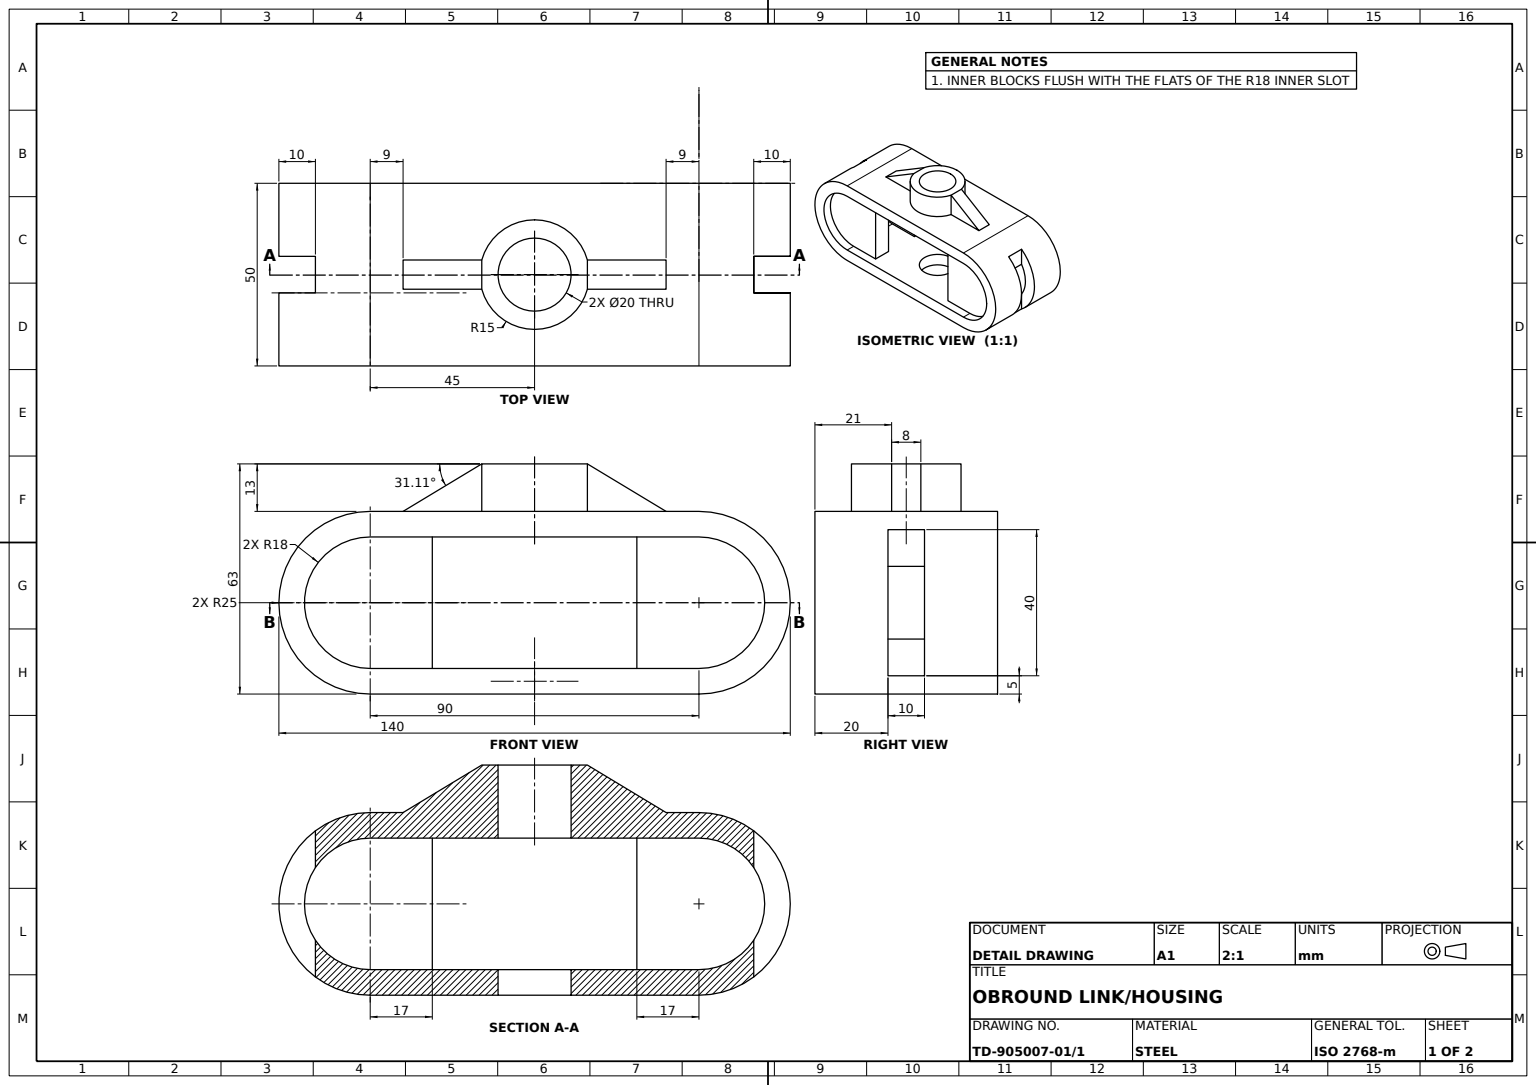
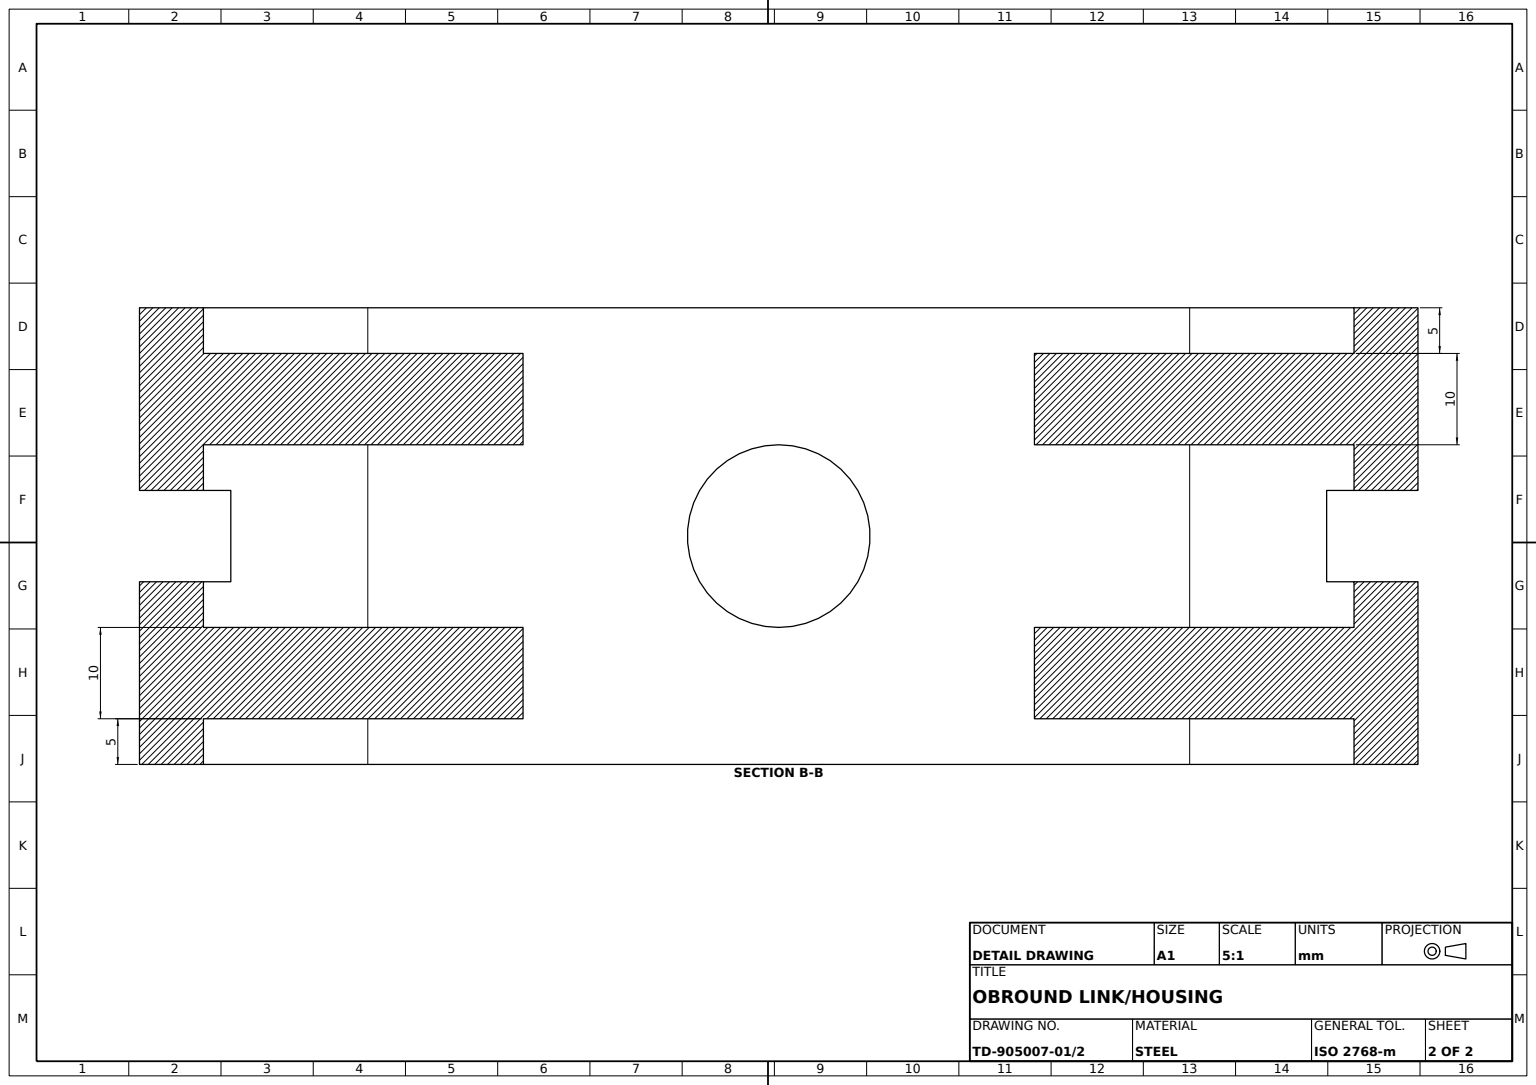
ISO-10303-21;
HEADER;
FILE_DESCRIPTION((''),'2;1');
FILE_NAME('','',(''),(''),'','','');
FILE_SCHEMA(('AUTOMOTIVE_DESIGN'));
ENDSEC;
DATA;
#1=APPLICATION_CONTEXT('');
#2=PRODUCT_CONTEXT('',#1,'mechanical');
#3=PRODUCT('','','',(#2));
#4=PRODUCT_DEFINITION_FORMATION('','',#3);
#5=PRODUCT_DEFINITION_CONTEXT('',#1,'design');
#6=PRODUCT_DEFINITION('','',#4,#5);
#7=PRODUCT_DEFINITION_SHAPE('','',#6);
#8=(LENGTH_UNIT()NAMED_UNIT(*)SI_UNIT(.MILLI.,.METRE.));
#9=(NAMED_UNIT(*)PLANE_ANGLE_UNIT()SI_UNIT($,.RADIAN.));
#10=(NAMED_UNIT(*)SI_UNIT($,.STERADIAN.)SOLID_ANGLE_UNIT());
#11=UNCERTAINTY_MEASURE_WITH_UNIT(LENGTH_MEASURE(1.E-05),#8,'distance_accuracy_value','');
#12=(GEOMETRIC_REPRESENTATION_CONTEXT(3)GLOBAL_UNCERTAINTY_ASSIGNED_CONTEXT((#11))GLOBAL_UNIT_ASSIGNED_CONTEXT((#8,#9,#10))REPRESENTATION_CONTEXT('',''));
#13=CARTESIAN_POINT('',(-15.,9.949874,-20.));
#14=VERTEX_POINT('',#13);
#15=CARTESIAN_POINT('',(-15.,20.,-20.));
#16=VERTEX_POINT('',#15);
#17=CARTESIAN_POINT('',(-15.,-25.,-20.));
#18=DIRECTION('',(0.,1.,0.));
#19=VECTOR('',#18,1000.);
#20=LINE('',#17,#19);
#21=EDGE_CURVE('',#14,#16,#20,.T.);
#22=ORIENTED_EDGE('',*,*,#21,.F.);
#23=CARTESIAN_POINT('',(-15.,-9.949874,-20.));
#24=VERTEX_POINT('',#23);
#25=CARTESIAN_POINT('',(0.,0.,-20.));
#26=DIRECTION('',(0.,0.,-1.));
#27=DIRECTION('',(1.,0.,0.));
#28=AXIS2_PLACEMENT_3D('',#25,#26,#27);
#29=CIRCLE('',#28,18.);
#30=EDGE_CURVE('',#24,#14,#29,.T.);
#31=ORIENTED_EDGE('',*,*,#30,.F.);
#32=CARTESIAN_POINT('',(-15.,-20.,-20.));
#33=VERTEX_POINT('',#32);
#34=EDGE_CURVE('',#33,#24,#20,.T.);
#35=ORIENTED_EDGE('',*,*,#34,.F.);
#36=CIRCLE('',#28,25.);
#37=EDGE_CURVE('',#33,#16,#36,.T.);
#38=ORIENTED_EDGE('',*,*,#37,.T.);
#39=EDGE_LOOP('',(#22,#31,#35,#38));
#40=FACE_OUTER_BOUND('',#39,.T.);
#41=DIRECTION('',(0.,0.,1.));
#42=AXIS2_PLACEMENT_3D('',#17,#41,#27);
#43=PLANE('',#42);
#44=ADVANCED_FACE('',(#40),#43,.F.);
#45=CARTESIAN_POINT('',(-15.,-20.,-30.));
#46=VERTEX_POINT('',#45);
#47=CARTESIAN_POINT('',(-15.,-20.,-50.));
#48=VECTOR('',#41,1000.);
#49=LINE('',#47,#48);
#50=EDGE_CURVE('',#46,#33,#49,.T.);
#51=ORIENTED_EDGE('',*,*,#50,.T.);
#52=ORIENTED_EDGE('',*,*,#34,.T.);
#53=CARTESIAN_POINT('',(-15.,-9.949874,-30.));
#54=VERTEX_POINT('',#53);
#55=CARTESIAN_POINT('',(-15.,-9.949874,-50.));
#56=LINE('',#55,#48);
#57=EDGE_CURVE('',#54,#24,#56,.T.);
#58=ORIENTED_EDGE('',*,*,#57,.F.);
#59=CARTESIAN_POINT('',(-15.,-25.,-30.));
#60=LINE('',#59,#19);
#61=EDGE_CURVE('',#46,#54,#60,.T.);
#62=ORIENTED_EDGE('',*,*,#61,.F.);
#63=EDGE_LOOP('',(#51,#52,#58,#62));
#64=FACE_OUTER_BOUND('',#63,.T.);
#65=AXIS2_PLACEMENT_3D('',#59,#27,#26);
#66=PLANE('',#65);
#67=ADVANCED_FACE('',(#64),#66,.F.);
#68=CARTESIAN_POINT('',(108.,0.,-45.));
#69=VERTEX_POINT('',#68);
#70=CARTESIAN_POINT('',(90.,18.,-45.));
#71=VERTEX_POINT('',#70);
#72=CARTESIAN_POINT('',(90.,0.,-45.));
#73=DIRECTION('',(-1.,0.,0.));
#74=AXIS2_PLACEMENT_3D('',#72,#41,#73);
#75=CIRCLE('',#74,18.);
#76=EDGE_CURVE('',#69,#71,#75,.T.);
#77=ORIENTED_EDGE('',*,*,#76,.F.);
#78=CARTESIAN_POINT('',(90.,-18.,-45.));
#79=VERTEX_POINT('',#78);
#80=EDGE_CURVE('',#79,#69,#75,.T.);
#81=ORIENTED_EDGE('',*,*,#80,.F.);
#82=CARTESIAN_POINT('',(73.,-18.,-45.));
#83=VERTEX_POINT('',#82);
#84=VECTOR('',#27,1000.);
#85=LINE('',#78,#84);
#86=EDGE_CURVE('',#83,#79,#85,.T.);
#87=ORIENTED_EDGE('',*,*,#86,.F.);
#88=CARTESIAN_POINT('',(73.,18.,-45.));
#89=VERTEX_POINT('',#88);
#90=DIRECTION('',(0.,-1.,0.));
#91=VECTOR('',#90,1000.);
#92=LINE('',#82,#91);
#93=EDGE_CURVE('',#89,#83,#92,.T.);
#94=ORIENTED_EDGE('',*,*,#93,.F.);
#95=VECTOR('',#73,1000.);
#96=LINE('',#88,#95);
#97=EDGE_CURVE('',#71,#89,#96,.T.);
#98=ORIENTED_EDGE('',*,*,#97,.F.);
#99=EDGE_LOOP('',(#77,#81,#87,#94,#98));
#100=FACE_OUTER_BOUND('',#99,.T.);
#101=PLANE('',#74);
#102=ADVANCED_FACE('',(#100),#101,.F.);
#103=CARTESIAN_POINT('',(59.456832,25.,-29.));
#104=VERTEX_POINT('',#103);
#105=CARTESIAN_POINT('',(59.456832,38.,-29.));
#106=VERTEX_POINT('',#105);
#107=LINE('',#105,#19);
#108=EDGE_CURVE('',#104,#106,#107,.T.);
#109=ORIENTED_EDGE('',*,*,#108,.F.);
#110=CARTESIAN_POINT('',(45.,25.,-40.));
#111=VERTEX_POINT('',#110);
#112=CARTESIAN_POINT('',(45.,25.,-25.));
#113=AXIS2_PLACEMENT_3D('',#112,#18,#41);
#114=CIRCLE('',#113,15.);
#115=EDGE_CURVE('',#104,#111,#114,.T.);
#116=ORIENTED_EDGE('',*,*,#115,.T.);
#117=CARTESIAN_POINT('',(45.,38.,-40.));
#118=VERTEX_POINT('',#117);
#119=LINE('',#117,#91);
#120=EDGE_CURVE('',#118,#111,#119,.T.);
#121=ORIENTED_EDGE('',*,*,#120,.F.);
#122=CARTESIAN_POINT('',(45.,38.,-25.));
#123=AXIS2_PLACEMENT_3D('',#122,#18,#41);
#124=CIRCLE('',#123,15.);
#125=EDGE_CURVE('',#106,#118,#124,.T.);
#126=ORIENTED_EDGE('',*,*,#125,.F.);
#127=EDGE_LOOP('',(#109,#116,#121,#126));
#128=FACE_OUTER_BOUND('',#127,.T.);
#129=AXIS2_PLACEMENT_3D('',#122,#90,#26);
#130=CYLINDRICAL_SURFACE('',#129,15.);
#131=ADVANCED_FACE('',(#128),#130,.T.);
#132=CARTESIAN_POINT('',(90.,-18.,-5.));
#133=VERTEX_POINT('',#132);
#134=CARTESIAN_POINT('',(90.,-18.,0.));
#135=VERTEX_POINT('',#134);
#136=CARTESIAN_POINT('',(90.,-18.,-50.));
#137=LINE('',#136,#48);
#138=EDGE_CURVE('',#133,#135,#137,.T.);
#139=ORIENTED_EDGE('',*,*,#138,.T.);
#140=CARTESIAN_POINT('',(108.,0.,0.));
#141=VERTEX_POINT('',#140);
#142=CARTESIAN_POINT('',(90.,0.,0.));
#143=AXIS2_PLACEMENT_3D('',#142,#41,#27);
#144=CIRCLE('',#143,18.);
#145=EDGE_CURVE('',#135,#141,#144,.T.);
#146=ORIENTED_EDGE('',*,*,#145,.T.);
#147=CARTESIAN_POINT('',(108.,0.,-5.));
#148=VERTEX_POINT('',#147);
#149=CARTESIAN_POINT('',(108.,0.,-50.));
#150=LINE('',#149,#48);
#151=EDGE_CURVE('',#148,#141,#150,.T.);
#152=ORIENTED_EDGE('',*,*,#151,.F.);
#153=CARTESIAN_POINT('',(90.,0.,-5.));
#154=AXIS2_PLACEMENT_3D('',#153,#41,#73);
#155=CIRCLE('',#154,18.);
#156=EDGE_CURVE('',#133,#148,#155,.T.);
#157=ORIENTED_EDGE('',*,*,#156,.F.);
#158=EDGE_LOOP('',(#139,#146,#152,#157));
#159=FACE_OUTER_BOUND('',#158,.T.);
#160=CARTESIAN_POINT('',(90.,0.,-50.));
#161=AXIS2_PLACEMENT_3D('',#160,#41,#27);
#162=CYLINDRICAL_SURFACE('',#161,18.);
#163=ADVANCED_FACE('',(#159),#162,.F.);
#164=CARTESIAN_POINT('',(90.,18.,-50.));
#165=VERTEX_POINT('',#164);
#166=CARTESIAN_POINT('',(0.,18.,-50.));
#167=VERTEX_POINT('',#166);
#168=LINE('',#166,#95);
#169=EDGE_CURVE('',#165,#167,#168,.T.);
#170=ORIENTED_EDGE('',*,*,#169,.T.);
#171=CARTESIAN_POINT('',(0.,-18.,-50.));
#172=VERTEX_POINT('',#171);
#173=CARTESIAN_POINT('',(0.,0.,-50.));
#174=AXIS2_PLACEMENT_3D('',#173,#41,#27);
#175=CIRCLE('',#174,18.);
#176=EDGE_CURVE('',#167,#172,#175,.T.);
#177=ORIENTED_EDGE('',*,*,#176,.T.);
#178=VERTEX_POINT('',#136);
#179=LINE('',#171,#84);
#180=EDGE_CURVE('',#172,#178,#179,.T.);
#181=ORIENTED_EDGE('',*,*,#180,.T.);
#182=VERTEX_POINT('',#149);
#183=CIRCLE('',#161,18.);
#184=EDGE_CURVE('',#178,#182,#183,.T.);
#185=ORIENTED_EDGE('',*,*,#184,.T.);
#186=EDGE_CURVE('',#182,#165,#183,.T.);
#187=ORIENTED_EDGE('',*,*,#186,.T.);
#188=EDGE_LOOP('',(#170,#177,#181,#185,#187));
#189=FACE_BOUND('',#188,.T.);
#190=CARTESIAN_POINT('',(90.,-25.,-50.));
#191=VERTEX_POINT('',#190);
#192=CARTESIAN_POINT('',(115.,0.,-50.));
#193=VERTEX_POINT('',#192);
#194=CIRCLE('',#161,25.);
#195=EDGE_CURVE('',#191,#193,#194,.T.);
#196=ORIENTED_EDGE('',*,*,#195,.F.);
#197=CARTESIAN_POINT('',(0.,-25.,-50.));
#198=VERTEX_POINT('',#197);
#199=LINE('',#197,#84);
#200=EDGE_CURVE('',#198,#191,#199,.T.);
#201=ORIENTED_EDGE('',*,*,#200,.F.);
#202=CARTESIAN_POINT('',(0.,25.,-50.));
#203=VERTEX_POINT('',#202);
#204=CIRCLE('',#174,25.);
#205=EDGE_CURVE('',#203,#198,#204,.T.);
#206=ORIENTED_EDGE('',*,*,#205,.F.);
#207=CARTESIAN_POINT('',(90.,25.,-50.));
#208=VERTEX_POINT('',#207);
#209=LINE('',#202,#95);
#210=EDGE_CURVE('',#208,#203,#209,.T.);
#211=ORIENTED_EDGE('',*,*,#210,.F.);
#212=EDGE_CURVE('',#193,#208,#194,.T.);
#213=ORIENTED_EDGE('',*,*,#212,.F.);
#214=EDGE_LOOP('',(#196,#201,#206,#211,#213));
#215=FACE_OUTER_BOUND('',#214,.T.);
#216=PLANE('',#174);
#217=ADVANCED_FACE('',(#189,#215),#216,.F.);
#218=CARTESIAN_POINT('',(115.,0.,-20.));
#219=VERTEX_POINT('',#218);
#220=CARTESIAN_POINT('',(105.,-20.,-20.));
#221=VERTEX_POINT('',#220);
#222=CARTESIAN_POINT('',(90.,0.,-20.));
#223=AXIS2_PLACEMENT_3D('',#222,#26,#27);
#224=CIRCLE('',#223,25.);
#225=EDGE_CURVE('',#219,#221,#224,.T.);
#226=ORIENTED_EDGE('',*,*,#225,.F.);
#227=CARTESIAN_POINT('',(115.,0.,0.));
#228=VERTEX_POINT('',#227);
#229=LINE('',#192,#48);
#230=EDGE_CURVE('',#219,#228,#229,.T.);
#231=ORIENTED_EDGE('',*,*,#230,.T.);
#232=CARTESIAN_POINT('',(90.,-25.,0.));
#233=VERTEX_POINT('',#232);
#234=CIRCLE('',#143,25.);
#235=EDGE_CURVE('',#233,#228,#234,.T.);
#236=ORIENTED_EDGE('',*,*,#235,.F.);
#237=LINE('',#190,#48);
#238=EDGE_CURVE('',#191,#233,#237,.T.);
#239=ORIENTED_EDGE('',*,*,#238,.F.);
#240=ORIENTED_EDGE('',*,*,#195,.T.);
#241=CARTESIAN_POINT('',(115.,0.,-30.));
#242=VERTEX_POINT('',#241);
#243=EDGE_CURVE('',#193,#242,#229,.T.);
#244=ORIENTED_EDGE('',*,*,#243,.T.);
#245=CARTESIAN_POINT('',(105.,-20.,-30.));
#246=VERTEX_POINT('',#245);
#247=CARTESIAN_POINT('',(90.,0.,-30.));
#248=AXIS2_PLACEMENT_3D('',#247,#41,#73);
#249=CIRCLE('',#248,25.);
#250=EDGE_CURVE('',#246,#242,#249,.T.);
#251=ORIENTED_EDGE('',*,*,#250,.F.);
#252=CARTESIAN_POINT('',(105.,-20.,-50.));
#253=VECTOR('',#26,1000.);
#254=LINE('',#252,#253);
#255=EDGE_CURVE('',#221,#246,#254,.T.);
#256=ORIENTED_EDGE('',*,*,#255,.F.);
#257=EDGE_LOOP('',(#226,#231,#236,#239,#240,#244,#251,#256));
#258=FACE_OUTER_BOUND('',#257,.T.);
#259=CYLINDRICAL_SURFACE('',#161,25.);
#260=ADVANCED_FACE('',(#258),#259,.T.);
#261=CARTESIAN_POINT('',(30.543168,38.,-29.));
#262=VERTEX_POINT('',#261);
#263=EDGE_CURVE('',#118,#262,#124,.T.);
#264=ORIENTED_EDGE('',*,*,#263,.T.);
#265=CARTESIAN_POINT('',(30.543168,38.,-21.));
#266=VERTEX_POINT('',#265);
#267=CARTESIAN_POINT('',(30.543168,38.,207.073716));
#268=LINE('',#267,#253);
#269=EDGE_CURVE('',#266,#262,#268,.T.);
#270=ORIENTED_EDGE('',*,*,#269,.F.);
#271=CARTESIAN_POINT('',(59.456832,38.,-21.));
#272=VERTEX_POINT('',#271);
#273=EDGE_CURVE('',#266,#272,#124,.T.);
#274=ORIENTED_EDGE('',*,*,#273,.T.);
#275=CARTESIAN_POINT('',(59.456832,38.,180.823716));
#276=LINE('',#275,#253);
#277=EDGE_CURVE('',#272,#106,#276,.T.);
#278=ORIENTED_EDGE('',*,*,#277,.T.);
#279=ORIENTED_EDGE('',*,*,#125,.T.);
#280=EDGE_LOOP('',(#264,#270,#274,#278,#279));
#281=FACE_OUTER_BOUND('',#280,.T.);
#282=CARTESIAN_POINT('',(45.,38.,-35.));
#283=VERTEX_POINT('',#282);
#284=CARTESIAN_POINT('',(45.,38.,-15.));
#285=VERTEX_POINT('',#284);
#286=CIRCLE('',#123,10.);
#287=EDGE_CURVE('',#283,#285,#286,.T.);
#288=ORIENTED_EDGE('',*,*,#287,.F.);
#289=EDGE_CURVE('',#285,#283,#286,.T.);
#290=ORIENTED_EDGE('',*,*,#289,.F.);
#291=EDGE_LOOP('',(#288,#290));
#292=FACE_BOUND('',#291,.T.);
#293=PLANE('',#123);
#294=ADVANCED_FACE('',(#281,#292),#293,.T.);
#295=CARTESIAN_POINT('',(9.,25.,-29.));
#296=VERTEX_POINT('',#295);
#297=CARTESIAN_POINT('',(86.706139,71.89096,-29.));
#298=DIRECTION('',(0.856190956,0.516659508,0.));
#299=VECTOR('',#298,1000.);
#300=LINE('',#297,#299);
#301=EDGE_CURVE('',#296,#262,#300,.T.);
#302=ORIENTED_EDGE('',*,*,#301,.T.);
#303=CARTESIAN_POINT('',(30.543168,25.,-29.));
#304=VERTEX_POINT('',#303);
#305=LINE('',#261,#19);
#306=EDGE_CURVE('',#304,#262,#305,.T.);
#307=ORIENTED_EDGE('',*,*,#306,.F.);
#308=CARTESIAN_POINT('',(115.002,25.,-29.));
#309=LINE('',#308,#95);
#310=EDGE_CURVE('',#304,#296,#309,.T.);
#311=ORIENTED_EDGE('',*,*,#310,.T.);
#312=EDGE_LOOP('',(#302,#307,#311));
#313=FACE_OUTER_BOUND('',#312,.T.);
#314=AXIS2_PLACEMENT_3D('',#308,#41,#90);
#315=PLANE('',#314);
#316=ADVANCED_FACE('',(#313),#315,.F.);
#317=CARTESIAN_POINT('',(45.,18.,-35.));
#318=VERTEX_POINT('',#317);
#319=CARTESIAN_POINT('',(45.,-25.,-35.));
#320=LINE('',#319,#19);
#321=EDGE_CURVE('',#318,#283,#320,.T.);
#322=ORIENTED_EDGE('',*,*,#321,.F.);
#323=CARTESIAN_POINT('',(45.,18.,-15.));
#324=VERTEX_POINT('',#323);
#325=CARTESIAN_POINT('',(45.,18.,-25.));
#326=AXIS2_PLACEMENT_3D('',#325,#18,#41);
#327=CIRCLE('',#326,10.);
#328=EDGE_CURVE('',#324,#318,#327,.T.);
#329=ORIENTED_EDGE('',*,*,#328,.F.);
#330=CARTESIAN_POINT('',(45.,-25.,-15.));
#331=LINE('',#330,#19);
#332=EDGE_CURVE('',#324,#285,#331,.T.);
#333=ORIENTED_EDGE('',*,*,#332,.T.);
#334=ORIENTED_EDGE('',*,*,#289,.T.);
#335=EDGE_LOOP('',(#322,#329,#333,#334));
#336=FACE_OUTER_BOUND('',#335,.T.);
#337=CARTESIAN_POINT('',(45.,-25.,-25.));
#338=AXIS2_PLACEMENT_3D('',#337,#18,#41);
#339=CYLINDRICAL_SURFACE('',#338,10.);
#340=ADVANCED_FACE('',(#336),#339,.F.);
#341=CARTESIAN_POINT('',(-15.,9.949874,-30.));
#342=VERTEX_POINT('',#341);
#343=CARTESIAN_POINT('',(-15.,9.949874,-50.));
#344=LINE('',#343,#253);
#345=EDGE_CURVE('',#14,#342,#344,.T.);
#346=ORIENTED_EDGE('',*,*,#345,.F.);
#347=ORIENTED_EDGE('',*,*,#21,.T.);
#348=CARTESIAN_POINT('',(-15.,20.,-30.));
#349=VERTEX_POINT('',#348);
#350=CARTESIAN_POINT('',(-15.,20.,-50.));
#351=LINE('',#350,#253);
#352=EDGE_CURVE('',#16,#349,#351,.T.);
#353=ORIENTED_EDGE('',*,*,#352,.T.);
#354=EDGE_CURVE('',#342,#349,#60,.T.);
#355=ORIENTED_EDGE('',*,*,#354,.F.);
#356=EDGE_LOOP('',(#346,#347,#353,#355));
#357=FACE_OUTER_BOUND('',#356,.T.);
#358=ADVANCED_FACE('',(#357),#66,.F.);
#359=EDGE_CURVE('',#111,#304,#114,.T.);
#360=ORIENTED_EDGE('',*,*,#359,.F.);
#361=ORIENTED_EDGE('',*,*,#115,.F.);
#362=CARTESIAN_POINT('',(81.,25.,-29.));
#363=VERTEX_POINT('',#362);
#364=CARTESIAN_POINT('',(-25.002,25.,-29.));
#365=LINE('',#364,#84);
#366=EDGE_CURVE('',#104,#363,#365,.T.);
#367=ORIENTED_EDGE('',*,*,#366,.T.);
#368=CARTESIAN_POINT('',(81.,25.,-21.));
#369=VERTEX_POINT('',#368);
#370=LINE('',#362,#253);
#371=EDGE_CURVE('',#369,#363,#370,.T.);
#372=ORIENTED_EDGE('',*,*,#371,.F.);
#373=CARTESIAN_POINT('',(59.456832,25.,-21.));
#374=VERTEX_POINT('',#373);
#375=CARTESIAN_POINT('',(-25.002,25.,-21.));
#376=LINE('',#375,#84);
#377=EDGE_CURVE('',#374,#369,#376,.T.);
#378=ORIENTED_EDGE('',*,*,#377,.F.);
#379=CARTESIAN_POINT('',(30.543168,25.,-21.));
#380=VERTEX_POINT('',#379);
#381=EDGE_CURVE('',#380,#374,#114,.T.);
#382=ORIENTED_EDGE('',*,*,#381,.F.);
#383=CARTESIAN_POINT('',(9.,25.,-21.));
#384=VERTEX_POINT('',#383);
#385=CARTESIAN_POINT('',(115.002,25.,-21.));
#386=LINE('',#385,#95);
#387=EDGE_CURVE('',#380,#384,#386,.T.);
#388=ORIENTED_EDGE('',*,*,#387,.T.);
#389=LINE('',#295,#253);
#390=EDGE_CURVE('',#384,#296,#389,.T.);
#391=ORIENTED_EDGE('',*,*,#390,.T.);
#392=ORIENTED_EDGE('',*,*,#310,.F.);
#393=EDGE_LOOP('',(#360,#361,#367,#372,#378,#382,#388,#391,#392));
#394=FACE_BOUND('',#393,.T.);
#395=CARTESIAN_POINT('',(90.,25.,0.));
#396=VERTEX_POINT('',#395);
#397=LINE('',#207,#48);
#398=EDGE_CURVE('',#208,#396,#397,.T.);
#399=ORIENTED_EDGE('',*,*,#398,.F.);
#400=ORIENTED_EDGE('',*,*,#210,.T.);
#401=CARTESIAN_POINT('',(0.,25.,0.));
#402=VERTEX_POINT('',#401);
#403=LINE('',#202,#48);
#404=EDGE_CURVE('',#203,#402,#403,.T.);
#405=ORIENTED_EDGE('',*,*,#404,.T.);
#406=LINE('',#401,#95);
#407=EDGE_CURVE('',#396,#402,#406,.T.);
#408=ORIENTED_EDGE('',*,*,#407,.F.);
#409=EDGE_LOOP('',(#399,#400,#405,#408));
#410=FACE_OUTER_BOUND('',#409,.T.);
#411=AXIS2_PLACEMENT_3D('',#202,#18,#41);
#412=PLANE('',#411);
#413=ADVANCED_FACE('',(#394,#410),#412,.T.);
#414=CARTESIAN_POINT('',(45.,-18.,-15.));
#415=VERTEX_POINT('',#414);
#416=CARTESIAN_POINT('',(45.,-18.,-35.));
#417=VERTEX_POINT('',#416);
#418=CARTESIAN_POINT('',(45.,-18.,-25.));
#419=AXIS2_PLACEMENT_3D('',#418,#90,#26);
#420=CIRCLE('',#419,10.);
#421=EDGE_CURVE('',#415,#417,#420,.T.);
#422=ORIENTED_EDGE('',*,*,#421,.T.);
#423=EDGE_CURVE('',#417,#415,#420,.T.);
#424=ORIENTED_EDGE('',*,*,#423,.T.);
#425=EDGE_LOOP('',(#422,#424));
#426=FACE_BOUND('',#425,.T.);
#427=CARTESIAN_POINT('',(73.,-18.,-15.));
#428=VERTEX_POINT('',#427);
#429=CARTESIAN_POINT('',(90.,-18.,-15.));
#430=VERTEX_POINT('',#429);
#431=LINE('',#429,#84);
#432=EDGE_CURVE('',#428,#430,#431,.T.);
#433=ORIENTED_EDGE('',*,*,#432,.T.);
#434=CARTESIAN_POINT('',(90.,-18.,-35.));
#435=VERTEX_POINT('',#434);
#436=EDGE_CURVE('',#435,#430,#137,.T.);
#437=ORIENTED_EDGE('',*,*,#436,.F.);
#438=CARTESIAN_POINT('',(73.,-18.,-35.));
#439=VERTEX_POINT('',#438);
#440=LINE('',#434,#84);
#441=EDGE_CURVE('',#439,#435,#440,.T.);
#442=ORIENTED_EDGE('',*,*,#441,.F.);
#443=LINE('',#438,#253);
#444=EDGE_CURVE('',#439,#83,#443,.T.);
#445=ORIENTED_EDGE('',*,*,#444,.T.);
#446=ORIENTED_EDGE('',*,*,#86,.T.);
#447=EDGE_CURVE('',#178,#79,#137,.T.);
#448=ORIENTED_EDGE('',*,*,#447,.F.);
#449=ORIENTED_EDGE('',*,*,#180,.F.);
#450=CARTESIAN_POINT('',(0.,-18.,-45.));
#451=VERTEX_POINT('',#450);
#452=LINE('',#171,#48);
#453=EDGE_CURVE('',#172,#451,#452,.T.);
#454=ORIENTED_EDGE('',*,*,#453,.T.);
#455=CARTESIAN_POINT('',(17.,-18.,-45.));
#456=VERTEX_POINT('',#455);
#457=LINE('',#455,#84);
#458=EDGE_CURVE('',#451,#456,#457,.T.);
#459=ORIENTED_EDGE('',*,*,#458,.T.);
#460=CARTESIAN_POINT('',(17.,-18.,-35.));
#461=VERTEX_POINT('',#460);
#462=LINE('',#460,#253);
#463=EDGE_CURVE('',#461,#456,#462,.T.);
#464=ORIENTED_EDGE('',*,*,#463,.F.);
#465=CARTESIAN_POINT('',(0.,-18.,-35.));
#466=VERTEX_POINT('',#465);
#467=LINE('',#460,#84);
#468=EDGE_CURVE('',#466,#461,#467,.T.);
#469=ORIENTED_EDGE('',*,*,#468,.F.);
#470=CARTESIAN_POINT('',(0.,-18.,-15.));
#471=VERTEX_POINT('',#470);
#472=EDGE_CURVE('',#466,#471,#452,.T.);
#473=ORIENTED_EDGE('',*,*,#472,.T.);
#474=CARTESIAN_POINT('',(17.,-18.,-15.));
#475=VERTEX_POINT('',#474);
#476=LINE('',#474,#84);
#477=EDGE_CURVE('',#471,#475,#476,.T.);
#478=ORIENTED_EDGE('',*,*,#477,.T.);
#479=CARTESIAN_POINT('',(17.,-18.,-5.));
#480=VERTEX_POINT('',#479);
#481=LINE('',#474,#48);
#482=EDGE_CURVE('',#475,#480,#481,.T.);
#483=ORIENTED_EDGE('',*,*,#482,.T.);
#484=CARTESIAN_POINT('',(0.,-18.,-5.));
#485=VERTEX_POINT('',#484);
#486=LINE('',#479,#84);
#487=EDGE_CURVE('',#485,#480,#486,.T.);
#488=ORIENTED_EDGE('',*,*,#487,.F.);
#489=CARTESIAN_POINT('',(0.,-18.,0.));
#490=VERTEX_POINT('',#489);
#491=EDGE_CURVE('',#485,#490,#452,.T.);
#492=ORIENTED_EDGE('',*,*,#491,.T.);
#493=LINE('',#489,#84);
#494=EDGE_CURVE('',#490,#135,#493,.T.);
#495=ORIENTED_EDGE('',*,*,#494,.T.);
#496=ORIENTED_EDGE('',*,*,#138,.F.);
#497=CARTESIAN_POINT('',(73.,-18.,-5.));
#498=VERTEX_POINT('',#497);
#499=LINE('',#132,#84);
#500=EDGE_CURVE('',#498,#133,#499,.T.);
#501=ORIENTED_EDGE('',*,*,#500,.F.);
#502=LINE('',#427,#48);
#503=EDGE_CURVE('',#428,#498,#502,.T.);
#504=ORIENTED_EDGE('',*,*,#503,.F.);
#505=EDGE_LOOP('',(#433,#437,#442,#445,#446,#448,#449,#454,#459,#464,#469,#473,#478,#483,#488,#492,#495,#496,#501,#504));
#506=FACE_OUTER_BOUND('',#505,.T.);
#507=AXIS2_PLACEMENT_3D('',#171,#90,#26);
#508=PLANE('',#507);
#509=ADVANCED_FACE('',(#426,#506),#508,.F.);
#510=CARTESIAN_POINT('',(0.,18.,-45.));
#511=VERTEX_POINT('',#510);
#512=LINE('',#166,#48);
#513=EDGE_CURVE('',#167,#511,#512,.T.);
#514=ORIENTED_EDGE('',*,*,#513,.T.);
#515=CARTESIAN_POINT('',(0.,0.,-45.));
#516=AXIS2_PLACEMENT_3D('',#515,#41,#27);
#517=CIRCLE('',#516,18.);
#518=EDGE_CURVE('',#511,#451,#517,.T.);
#519=ORIENTED_EDGE('',*,*,#518,.T.);
#520=ORIENTED_EDGE('',*,*,#453,.F.);
#521=ORIENTED_EDGE('',*,*,#176,.F.);
#522=EDGE_LOOP('',(#514,#519,#520,#521));
#523=FACE_OUTER_BOUND('',#522,.T.);
#524=CYLINDRICAL_SURFACE('',#174,18.);
#525=ADVANCED_FACE('',(#523),#524,.F.);
#526=ORIENTED_EDGE('',*,*,#277,.F.);
#527=DIRECTION('',(0.856190956,-0.516659508,0.));
#528=VECTOR('',#527,1000.);
#529=LINE('',#271,#528);
#530=EDGE_CURVE('',#272,#369,#529,.T.);
#531=ORIENTED_EDGE('',*,*,#530,.T.);
#532=ORIENTED_EDGE('',*,*,#371,.T.);
#533=CARTESIAN_POINT('',(3.293861,71.89096,-29.));
#534=LINE('',#533,#528);
#535=EDGE_CURVE('',#106,#363,#534,.T.);
#536=ORIENTED_EDGE('',*,*,#535,.F.);
#537=EDGE_LOOP('',(#526,#531,#532,#536));
#538=FACE_OUTER_BOUND('',#537,.T.);
#539=DIRECTION('',(0.516659508,0.856190956,0.));
#540=DIRECTION('',(-0.856190956,0.516659508,0.));
#541=AXIS2_PLACEMENT_3D('',#275,#539,#540);
#542=PLANE('',#541);
#543=ADVANCED_FACE('',(#538),#542,.T.);
#544=CARTESIAN_POINT('',(17.,18.,-15.));
#545=VERTEX_POINT('',#544);
#546=CARTESIAN_POINT('',(0.,18.,-15.));
#547=VERTEX_POINT('',#546);
#548=LINE('',#544,#95);
#549=EDGE_CURVE('',#545,#547,#548,.T.);
#550=ORIENTED_EDGE('',*,*,#549,.F.);
#551=LINE('',#474,#19);
#552=EDGE_CURVE('',#475,#545,#551,.T.);
#553=ORIENTED_EDGE('',*,*,#552,.F.);
#554=ORIENTED_EDGE('',*,*,#477,.F.);
#555=CARTESIAN_POINT('',(0.,0.,-15.));
#556=AXIS2_PLACEMENT_3D('',#555,#41,#27);
#557=CIRCLE('',#556,18.);
#558=EDGE_CURVE('',#547,#471,#557,.T.);
#559=ORIENTED_EDGE('',*,*,#558,.F.);
#560=EDGE_LOOP('',(#550,#553,#554,#559));
#561=FACE_OUTER_BOUND('',#560,.T.);
#562=PLANE('',#556);
#563=ADVANCED_FACE('',(#561),#562,.F.);
#564=CARTESIAN_POINT('',(105.,-9.949874,-20.));
#565=VERTEX_POINT('',#564);
#566=CARTESIAN_POINT('',(105.,-9.949874,-30.));
#567=VERTEX_POINT('',#566);
#568=CARTESIAN_POINT('',(105.,-9.949874,-50.));
#569=LINE('',#568,#253);
#570=EDGE_CURVE('',#565,#567,#569,.T.);
#571=ORIENTED_EDGE('',*,*,#570,.F.);
#572=CARTESIAN_POINT('',(105.,-25.,-20.));
#573=LINE('',#572,#19);
#574=EDGE_CURVE('',#221,#565,#573,.T.);
#575=ORIENTED_EDGE('',*,*,#574,.F.);
#576=ORIENTED_EDGE('',*,*,#255,.T.);
#577=CARTESIAN_POINT('',(105.,-25.,-30.));
#578=LINE('',#577,#19);
#579=EDGE_CURVE('',#246,#567,#578,.T.);
#580=ORIENTED_EDGE('',*,*,#579,.T.);
#581=EDGE_LOOP('',(#571,#575,#576,#580));
#582=FACE_OUTER_BOUND('',#581,.T.);
#583=AXIS2_PLACEMENT_3D('',#577,#73,#41);
#584=PLANE('',#583);
#585=ADVANCED_FACE('',(#582),#584,.F.);
#586=ORIENTED_EDGE('',*,*,#487,.T.);
#587=CARTESIAN_POINT('',(17.,18.,-5.));
#588=VERTEX_POINT('',#587);
#589=LINE('',#479,#19);
#590=EDGE_CURVE('',#480,#588,#589,.T.);
#591=ORIENTED_EDGE('',*,*,#590,.T.);
#592=CARTESIAN_POINT('',(0.,18.,-5.));
#593=VERTEX_POINT('',#592);
#594=LINE('',#587,#95);
#595=EDGE_CURVE('',#588,#593,#594,.T.);
#596=ORIENTED_EDGE('',*,*,#595,.T.);
#597=CARTESIAN_POINT('',(0.,0.,-5.));
#598=AXIS2_PLACEMENT_3D('',#597,#41,#27);
#599=CIRCLE('',#598,18.);
#600=EDGE_CURVE('',#593,#485,#599,.T.);
#601=ORIENTED_EDGE('',*,*,#600,.T.);
#602=EDGE_LOOP('',(#586,#591,#596,#601));
#603=FACE_OUTER_BOUND('',#602,.T.);
#604=PLANE('',#598);
#605=ADVANCED_FACE('',(#603),#604,.T.);
#606=ORIENTED_EDGE('',*,*,#432,.F.);
#607=CARTESIAN_POINT('',(73.,18.,-15.));
#608=VERTEX_POINT('',#607);
#609=LINE('',#427,#91);
#610=EDGE_CURVE('',#608,#428,#609,.T.);
#611=ORIENTED_EDGE('',*,*,#610,.F.);
#612=CARTESIAN_POINT('',(90.,18.,-15.));
#613=VERTEX_POINT('',#612);
#614=LINE('',#607,#95);
#615=EDGE_CURVE('',#613,#608,#614,.T.);
#616=ORIENTED_EDGE('',*,*,#615,.F.);
#617=CARTESIAN_POINT('',(108.,0.,-15.));
#618=VERTEX_POINT('',#617);
#619=CARTESIAN_POINT('',(90.,0.,-15.));
#620=AXIS2_PLACEMENT_3D('',#619,#41,#73);
#621=CIRCLE('',#620,18.);
#622=EDGE_CURVE('',#618,#613,#621,.T.);
#623=ORIENTED_EDGE('',*,*,#622,.F.);
#624=EDGE_CURVE('',#430,#618,#621,.T.);
#625=ORIENTED_EDGE('',*,*,#624,.F.);
#626=EDGE_LOOP('',(#606,#611,#616,#623,#625));
#627=FACE_OUTER_BOUND('',#626,.T.);
#628=AXIS2_PLACEMENT_3D('',#619,#26,#73);
#629=PLANE('',#628);
#630=ADVANCED_FACE('',(#627),#629,.T.);
#631=ORIENTED_EDGE('',*,*,#590,.F.);
#632=ORIENTED_EDGE('',*,*,#482,.F.);
#633=ORIENTED_EDGE('',*,*,#552,.T.);
#634=LINE('',#544,#48);
#635=EDGE_CURVE('',#545,#588,#634,.T.);
#636=ORIENTED_EDGE('',*,*,#635,.T.);
#637=EDGE_LOOP('',(#631,#632,#633,#636));
#638=FACE_OUTER_BOUND('',#637,.T.);
#639=AXIS2_PLACEMENT_3D('',#474,#27,#18);
#640=PLANE('',#639);
#641=ADVANCED_FACE('',(#638),#640,.T.);
#642=VERTEX_POINT('',#319);
#643=EDGE_CURVE('',#642,#417,#320,.T.);
#644=ORIENTED_EDGE('',*,*,#643,.F.);
#645=VERTEX_POINT('',#330);
#646=CIRCLE('',#338,10.);
#647=EDGE_CURVE('',#645,#642,#646,.T.);
#648=ORIENTED_EDGE('',*,*,#647,.F.);
#649=EDGE_CURVE('',#645,#415,#331,.T.);
#650=ORIENTED_EDGE('',*,*,#649,.T.);
#651=ORIENTED_EDGE('',*,*,#423,.F.);
#652=EDGE_LOOP('',(#644,#648,#650,#651));
#653=FACE_OUTER_BOUND('',#652,.T.);
#654=ADVANCED_FACE('',(#653),#339,.F.);
#655=ORIENTED_EDGE('',*,*,#184,.F.);
#656=ORIENTED_EDGE('',*,*,#447,.T.);
#657=ORIENTED_EDGE('',*,*,#80,.T.);
#658=EDGE_CURVE('',#182,#69,#150,.T.);
#659=ORIENTED_EDGE('',*,*,#658,.F.);
#660=EDGE_LOOP('',(#655,#656,#657,#659));
#661=FACE_OUTER_BOUND('',#660,.T.);
#662=ADVANCED_FACE('',(#661),#162,.F.);
#663=LINE('',#271,#91);
#664=EDGE_CURVE('',#272,#374,#663,.T.);
#665=ORIENTED_EDGE('',*,*,#664,.T.);
#666=ORIENTED_EDGE('',*,*,#377,.T.);
#667=ORIENTED_EDGE('',*,*,#530,.F.);
#668=EDGE_LOOP('',(#665,#666,#667));
#669=FACE_OUTER_BOUND('',#668,.T.);
#670=AXIS2_PLACEMENT_3D('',#375,#41,#27);
#671=PLANE('',#670);
#672=ADVANCED_FACE('',(#669),#671,.T.);
#673=ORIENTED_EDGE('',*,*,#108,.T.);
#674=ORIENTED_EDGE('',*,*,#535,.T.);
#675=ORIENTED_EDGE('',*,*,#366,.F.);
#676=EDGE_LOOP('',(#673,#674,#675));
#677=FACE_OUTER_BOUND('',#676,.T.);
#678=AXIS2_PLACEMENT_3D('',#364,#26,#18);
#679=PLANE('',#678);
#680=ADVANCED_FACE('',(#677),#679,.T.);
#681=ORIENTED_EDGE('',*,*,#574,.T.);
#682=CARTESIAN_POINT('',(108.,0.,-20.));
#683=VERTEX_POINT('',#682);
#684=CIRCLE('',#223,18.);
#685=EDGE_CURVE('',#683,#565,#684,.T.);
#686=ORIENTED_EDGE('',*,*,#685,.F.);
#687=CARTESIAN_POINT('',(105.,9.949874,-20.));
#688=VERTEX_POINT('',#687);
#689=EDGE_CURVE('',#688,#683,#684,.T.);
#690=ORIENTED_EDGE('',*,*,#689,.F.);
#691=CARTESIAN_POINT('',(105.,20.,-20.));
#692=VERTEX_POINT('',#691);
#693=EDGE_CURVE('',#688,#692,#573,.T.);
#694=ORIENTED_EDGE('',*,*,#693,.T.);
#695=EDGE_CURVE('',#692,#219,#224,.T.);
#696=ORIENTED_EDGE('',*,*,#695,.T.);
#697=ORIENTED_EDGE('',*,*,#225,.T.);
#698=EDGE_LOOP('',(#681,#686,#690,#694,#696,#697));
#699=FACE_OUTER_BOUND('',#698,.T.);
#700=AXIS2_PLACEMENT_3D('',#572,#41,#27);
#701=PLANE('',#700);
#702=ADVANCED_FACE('',(#699),#701,.F.);
#703=ORIENTED_EDGE('',*,*,#301,.F.);
#704=ORIENTED_EDGE('',*,*,#390,.F.);
#705=LINE('',#265,#299);
#706=EDGE_CURVE('',#384,#266,#705,.T.);
#707=ORIENTED_EDGE('',*,*,#706,.T.);
#708=ORIENTED_EDGE('',*,*,#269,.T.);
#709=EDGE_LOOP('',(#703,#704,#707,#708));
#710=FACE_OUTER_BOUND('',#709,.T.);
#711=DIRECTION('',(0.516659508,-0.856190956,0.));
#712=AXIS2_PLACEMENT_3D('',#267,#711,#298);
#713=PLANE('',#712);
#714=ADVANCED_FACE('',(#710),#713,.F.);
#715=ORIENTED_EDGE('',*,*,#549,.T.);
#716=CARTESIAN_POINT('',(0.,18.,-35.));
#717=VERTEX_POINT('',#716);
#718=EDGE_CURVE('',#717,#547,#512,.T.);
#719=ORIENTED_EDGE('',*,*,#718,.F.);
#720=CARTESIAN_POINT('',(17.,18.,-35.));
#721=VERTEX_POINT('',#720);
#722=LINE('',#720,#95);
#723=EDGE_CURVE('',#721,#717,#722,.T.);
#724=ORIENTED_EDGE('',*,*,#723,.F.);
#725=CARTESIAN_POINT('',(17.,18.,-45.));
#726=VERTEX_POINT('',#725);
#727=LINE('',#720,#253);
#728=EDGE_CURVE('',#721,#726,#727,.T.);
#729=ORIENTED_EDGE('',*,*,#728,.T.);
#730=LINE('',#725,#95);
#731=EDGE_CURVE('',#726,#511,#730,.T.);
#732=ORIENTED_EDGE('',*,*,#731,.T.);
#733=ORIENTED_EDGE('',*,*,#513,.F.);
#734=ORIENTED_EDGE('',*,*,#169,.F.);
#735=LINE('',#164,#48);
#736=EDGE_CURVE('',#165,#71,#735,.T.);
#737=ORIENTED_EDGE('',*,*,#736,.T.);
#738=ORIENTED_EDGE('',*,*,#97,.T.);
#739=CARTESIAN_POINT('',(73.,18.,-35.));
#740=VERTEX_POINT('',#739);
#741=LINE('',#739,#253);
#742=EDGE_CURVE('',#740,#89,#741,.T.);
#743=ORIENTED_EDGE('',*,*,#742,.F.);
#744=CARTESIAN_POINT('',(90.,18.,-35.));
#745=VERTEX_POINT('',#744);
#746=LINE('',#739,#95);
#747=EDGE_CURVE('',#745,#740,#746,.T.);
#748=ORIENTED_EDGE('',*,*,#747,.F.);
#749=EDGE_CURVE('',#745,#613,#735,.T.);
#750=ORIENTED_EDGE('',*,*,#749,.T.);
#751=ORIENTED_EDGE('',*,*,#615,.T.);
#752=CARTESIAN_POINT('',(73.,18.,-5.));
#753=VERTEX_POINT('',#752);
#754=LINE('',#607,#48);
#755=EDGE_CURVE('',#608,#753,#754,.T.);
#756=ORIENTED_EDGE('',*,*,#755,.T.);
#757=CARTESIAN_POINT('',(90.,18.,-5.));
#758=VERTEX_POINT('',#757);
#759=LINE('',#752,#95);
#760=EDGE_CURVE('',#758,#753,#759,.T.);
#761=ORIENTED_EDGE('',*,*,#760,.F.);
#762=CARTESIAN_POINT('',(90.,18.,0.));
#763=VERTEX_POINT('',#762);
#764=EDGE_CURVE('',#758,#763,#735,.T.);
#765=ORIENTED_EDGE('',*,*,#764,.T.);
#766=CARTESIAN_POINT('',(0.,18.,0.));
#767=VERTEX_POINT('',#766);
#768=LINE('',#766,#95);
#769=EDGE_CURVE('',#763,#767,#768,.T.);
#770=ORIENTED_EDGE('',*,*,#769,.T.);
#771=EDGE_CURVE('',#593,#767,#512,.T.);
#772=ORIENTED_EDGE('',*,*,#771,.F.);
#773=ORIENTED_EDGE('',*,*,#595,.F.);
#774=ORIENTED_EDGE('',*,*,#635,.F.);
#775=EDGE_LOOP('',(#715,#719,#724,#729,#732,#733,#734,#737,#738,#743,#748,#750,#751,#756,#761,#765,#770,#772,#773,#774));
#776=FACE_OUTER_BOUND('',#775,.T.);
#777=EDGE_CURVE('',#318,#324,#327,.T.);
#778=ORIENTED_EDGE('',*,*,#777,.T.);
#779=ORIENTED_EDGE('',*,*,#328,.T.);
#780=EDGE_LOOP('',(#778,#779));
#781=FACE_BOUND('',#780,.T.);
#782=AXIS2_PLACEMENT_3D('',#166,#18,#41);
#783=PLANE('',#782);
#784=ADVANCED_FACE('',(#776,#781),#783,.F.);
#785=ORIENTED_EDGE('',*,*,#723,.T.);
#786=CARTESIAN_POINT('',(0.,0.,-35.));
#787=AXIS2_PLACEMENT_3D('',#786,#41,#27);
#788=CIRCLE('',#787,18.);
#789=EDGE_CURVE('',#717,#466,#788,.T.);
#790=ORIENTED_EDGE('',*,*,#789,.T.);
#791=ORIENTED_EDGE('',*,*,#468,.T.);
#792=LINE('',#460,#19);
#793=EDGE_CURVE('',#461,#721,#792,.T.);
#794=ORIENTED_EDGE('',*,*,#793,.T.);
#795=EDGE_LOOP('',(#785,#790,#791,#794));
#796=FACE_OUTER_BOUND('',#795,.T.);
#797=AXIS2_PLACEMENT_3D('',#786,#26,#27);
#798=PLANE('',#797);
#799=ADVANCED_FACE('',(#796),#798,.F.);
#800=ORIENTED_EDGE('',*,*,#771,.T.);
#801=CARTESIAN_POINT('',(0.,0.,0.));
#802=AXIS2_PLACEMENT_3D('',#801,#41,#27);
#803=CIRCLE('',#802,18.);
#804=EDGE_CURVE('',#767,#490,#803,.T.);
#805=ORIENTED_EDGE('',*,*,#804,.T.);
#806=ORIENTED_EDGE('',*,*,#491,.F.);
#807=ORIENTED_EDGE('',*,*,#600,.F.);
#808=EDGE_LOOP('',(#800,#805,#806,#807));
#809=FACE_OUTER_BOUND('',#808,.T.);
#810=ADVANCED_FACE('',(#809),#524,.F.);
#811=ORIENTED_EDGE('',*,*,#643,.T.);
#812=ORIENTED_EDGE('',*,*,#421,.F.);
#813=ORIENTED_EDGE('',*,*,#649,.F.);
#814=EDGE_CURVE('',#642,#645,#646,.T.);
#815=ORIENTED_EDGE('',*,*,#814,.F.);
#816=EDGE_LOOP('',(#811,#812,#813,#815));
#817=FACE_OUTER_BOUND('',#816,.T.);
#818=ADVANCED_FACE('',(#817),#339,.F.);
#819=ORIENTED_EDGE('',*,*,#463,.T.);
#820=LINE('',#455,#19);
#821=EDGE_CURVE('',#456,#726,#820,.T.);
#822=ORIENTED_EDGE('',*,*,#821,.T.);
#823=ORIENTED_EDGE('',*,*,#728,.F.);
#824=ORIENTED_EDGE('',*,*,#793,.F.);
#825=EDGE_LOOP('',(#819,#822,#823,#824));
#826=FACE_OUTER_BOUND('',#825,.T.);
#827=AXIS2_PLACEMENT_3D('',#460,#73,#90);
#828=PLANE('',#827);
#829=ADVANCED_FACE('',(#826),#828,.F.);
#830=ORIENTED_EDGE('',*,*,#444,.F.);
#831=LINE('',#438,#91);
#832=EDGE_CURVE('',#740,#439,#831,.T.);
#833=ORIENTED_EDGE('',*,*,#832,.F.);
#834=ORIENTED_EDGE('',*,*,#742,.T.);
#835=ORIENTED_EDGE('',*,*,#93,.T.);
#836=EDGE_LOOP('',(#830,#833,#834,#835));
#837=FACE_OUTER_BOUND('',#836,.T.);
#838=AXIS2_PLACEMENT_3D('',#438,#27,#18);
#839=PLANE('',#838);
#840=ADVANCED_FACE('',(#837),#839,.F.);
#841=CARTESIAN_POINT('',(0.,-25.,0.));
#842=VERTEX_POINT('',#841);
#843=LINE('',#841,#84);
#844=EDGE_CURVE('',#842,#233,#843,.T.);
#845=ORIENTED_EDGE('',*,*,#844,.T.);
#846=ORIENTED_EDGE('',*,*,#235,.T.);
#847=EDGE_CURVE('',#228,#396,#234,.T.);
#848=ORIENTED_EDGE('',*,*,#847,.T.);
#849=ORIENTED_EDGE('',*,*,#407,.T.);
#850=CIRCLE('',#802,25.);
#851=EDGE_CURVE('',#402,#842,#850,.T.);
#852=ORIENTED_EDGE('',*,*,#851,.T.);
#853=EDGE_LOOP('',(#845,#846,#848,#849,#852));
#854=FACE_OUTER_BOUND('',#853,.T.);
#855=EDGE_CURVE('',#141,#763,#144,.T.);
#856=ORIENTED_EDGE('',*,*,#855,.F.);
#857=ORIENTED_EDGE('',*,*,#145,.F.);
#858=ORIENTED_EDGE('',*,*,#494,.F.);
#859=ORIENTED_EDGE('',*,*,#804,.F.);
#860=ORIENTED_EDGE('',*,*,#769,.F.);
#861=EDGE_LOOP('',(#856,#857,#858,#859,#860));
#862=FACE_BOUND('',#861,.T.);
#863=PLANE('',#802);
#864=ADVANCED_FACE('',(#854,#862),#863,.T.);
#865=ORIENTED_EDGE('',*,*,#695,.F.);
#866=CARTESIAN_POINT('',(105.,20.,-30.));
#867=VERTEX_POINT('',#866);
#868=CARTESIAN_POINT('',(105.,20.,-50.));
#869=LINE('',#868,#48);
#870=EDGE_CURVE('',#867,#692,#869,.T.);
#871=ORIENTED_EDGE('',*,*,#870,.F.);
#872=EDGE_CURVE('',#242,#867,#249,.T.);
#873=ORIENTED_EDGE('',*,*,#872,.F.);
#874=ORIENTED_EDGE('',*,*,#243,.F.);
#875=ORIENTED_EDGE('',*,*,#212,.T.);
#876=ORIENTED_EDGE('',*,*,#398,.T.);
#877=ORIENTED_EDGE('',*,*,#847,.F.);
#878=ORIENTED_EDGE('',*,*,#230,.F.);
#879=EDGE_LOOP('',(#865,#871,#873,#874,#875,#876,#877,#878));
#880=FACE_OUTER_BOUND('',#879,.T.);
#881=ADVANCED_FACE('',(#880),#259,.T.);
#882=ORIENTED_EDGE('',*,*,#387,.F.);
#883=LINE('',#265,#91);
#884=EDGE_CURVE('',#266,#380,#883,.T.);
#885=ORIENTED_EDGE('',*,*,#884,.F.);
#886=ORIENTED_EDGE('',*,*,#706,.F.);
#887=EDGE_LOOP('',(#882,#885,#886));
#888=FACE_OUTER_BOUND('',#887,.T.);
#889=AXIS2_PLACEMENT_3D('',#385,#26,#73);
#890=PLANE('',#889);
#891=ADVANCED_FACE('',(#888),#890,.F.);
#892=ORIENTED_EDGE('',*,*,#30,.T.);
#893=ORIENTED_EDGE('',*,*,#345,.T.);
#894=CARTESIAN_POINT('',(0.,0.,-30.));
#895=AXIS2_PLACEMENT_3D('',#894,#41,#73);
#896=CIRCLE('',#895,18.);
#897=EDGE_CURVE('',#342,#54,#896,.T.);
#898=ORIENTED_EDGE('',*,*,#897,.T.);
#899=ORIENTED_EDGE('',*,*,#57,.T.);
#900=EDGE_LOOP('',(#892,#893,#898,#899));
#901=FACE_BOUND('',#900,.T.);
#902=ORIENTED_EDGE('',*,*,#558,.T.);
#903=ORIENTED_EDGE('',*,*,#472,.F.);
#904=ORIENTED_EDGE('',*,*,#789,.F.);
#905=ORIENTED_EDGE('',*,*,#718,.T.);
#906=EDGE_LOOP('',(#902,#903,#904,#905));
#907=FACE_OUTER_BOUND('',#906,.T.);
#908=ADVANCED_FACE('',(#901,#907),#524,.F.);
#909=ORIENTED_EDGE('',*,*,#359,.T.);
#910=ORIENTED_EDGE('',*,*,#306,.T.);
#911=ORIENTED_EDGE('',*,*,#263,.F.);
#912=ORIENTED_EDGE('',*,*,#120,.T.);
#913=EDGE_LOOP('',(#909,#910,#911,#912));
#914=FACE_OUTER_BOUND('',#913,.T.);
#915=ADVANCED_FACE('',(#914),#130,.T.);
#916=ORIENTED_EDGE('',*,*,#381,.T.);
#917=ORIENTED_EDGE('',*,*,#664,.F.);
#918=ORIENTED_EDGE('',*,*,#273,.F.);
#919=ORIENTED_EDGE('',*,*,#884,.T.);
#920=EDGE_LOOP('',(#916,#917,#918,#919));
#921=FACE_OUTER_BOUND('',#920,.T.);
#922=ADVANCED_FACE('',(#921),#130,.T.);
#923=ORIENTED_EDGE('',*,*,#518,.F.);
#924=ORIENTED_EDGE('',*,*,#731,.F.);
#925=ORIENTED_EDGE('',*,*,#821,.F.);
#926=ORIENTED_EDGE('',*,*,#458,.F.);
#927=EDGE_LOOP('',(#923,#924,#925,#926));
#928=FACE_OUTER_BOUND('',#927,.T.);
#929=AXIS2_PLACEMENT_3D('',#515,#26,#27);
#930=PLANE('',#929);
#931=ADVANCED_FACE('',(#928),#930,.T.);
#932=ORIENTED_EDGE('',*,*,#287,.T.);
#933=ORIENTED_EDGE('',*,*,#332,.F.);
#934=ORIENTED_EDGE('',*,*,#777,.F.);
#935=ORIENTED_EDGE('',*,*,#321,.T.);
#936=EDGE_LOOP('',(#932,#933,#934,#935));
#937=FACE_OUTER_BOUND('',#936,.T.);
#938=ADVANCED_FACE('',(#937),#339,.F.);
#939=CARTESIAN_POINT('',(105.,9.949874,-30.));
#940=VERTEX_POINT('',#939);
#941=EDGE_CURVE('',#940,#867,#578,.T.);
#942=ORIENTED_EDGE('',*,*,#941,.T.);
#943=ORIENTED_EDGE('',*,*,#870,.T.);
#944=ORIENTED_EDGE('',*,*,#693,.F.);
#945=CARTESIAN_POINT('',(105.,9.949874,-50.));
#946=LINE('',#945,#48);
#947=EDGE_CURVE('',#940,#688,#946,.T.);
#948=ORIENTED_EDGE('',*,*,#947,.F.);
#949=EDGE_LOOP('',(#942,#943,#944,#948));
#950=FACE_OUTER_BOUND('',#949,.T.);
#951=ADVANCED_FACE('',(#950),#584,.F.);
#952=ORIENTED_EDGE('',*,*,#76,.T.);
#953=ORIENTED_EDGE('',*,*,#736,.F.);
#954=ORIENTED_EDGE('',*,*,#186,.F.);
#955=ORIENTED_EDGE('',*,*,#658,.T.);
#956=EDGE_LOOP('',(#952,#953,#954,#955));
#957=FACE_OUTER_BOUND('',#956,.T.);
#958=ADVANCED_FACE('',(#957),#162,.F.);
#959=ORIENTED_EDGE('',*,*,#354,.T.);
#960=CIRCLE('',#895,25.);
#961=EDGE_CURVE('',#349,#46,#960,.T.);
#962=ORIENTED_EDGE('',*,*,#961,.T.);
#963=ORIENTED_EDGE('',*,*,#61,.T.);
#964=ORIENTED_EDGE('',*,*,#897,.F.);
#965=EDGE_LOOP('',(#959,#962,#963,#964));
#966=FACE_OUTER_BOUND('',#965,.T.);
#967=AXIS2_PLACEMENT_3D('',#59,#26,#73);
#968=PLANE('',#967);
#969=ADVANCED_FACE('',(#966),#968,.F.);
#970=CARTESIAN_POINT('',(108.,0.,-35.));
#971=VERTEX_POINT('',#970);
#972=CARTESIAN_POINT('',(108.,0.,-30.));
#973=VERTEX_POINT('',#972);
#974=EDGE_CURVE('',#971,#973,#150,.T.);
#975=ORIENTED_EDGE('',*,*,#974,.F.);
#976=CARTESIAN_POINT('',(90.,0.,-35.));
#977=AXIS2_PLACEMENT_3D('',#976,#41,#73);
#978=CIRCLE('',#977,18.);
#979=EDGE_CURVE('',#435,#971,#978,.T.);
#980=ORIENTED_EDGE('',*,*,#979,.F.);
#981=ORIENTED_EDGE('',*,*,#436,.T.);
#982=ORIENTED_EDGE('',*,*,#624,.T.);
#983=EDGE_CURVE('',#683,#618,#150,.T.);
#984=ORIENTED_EDGE('',*,*,#983,.F.);
#985=ORIENTED_EDGE('',*,*,#685,.T.);
#986=ORIENTED_EDGE('',*,*,#570,.T.);
#987=CIRCLE('',#248,18.);
#988=EDGE_CURVE('',#567,#973,#987,.T.);
#989=ORIENTED_EDGE('',*,*,#988,.T.);
#990=EDGE_LOOP('',(#975,#980,#981,#982,#984,#985,#986,#989));
#991=FACE_OUTER_BOUND('',#990,.T.);
#992=ADVANCED_FACE('',(#991),#162,.F.);
#993=ORIENTED_EDGE('',*,*,#689,.T.);
#994=ORIENTED_EDGE('',*,*,#983,.T.);
#995=ORIENTED_EDGE('',*,*,#622,.T.);
#996=ORIENTED_EDGE('',*,*,#749,.F.);
#997=EDGE_CURVE('',#971,#745,#978,.T.);
#998=ORIENTED_EDGE('',*,*,#997,.F.);
#999=ORIENTED_EDGE('',*,*,#974,.T.);
#1000=EDGE_CURVE('',#973,#940,#987,.T.);
#1001=ORIENTED_EDGE('',*,*,#1000,.T.);
#1002=ORIENTED_EDGE('',*,*,#947,.T.);
#1003=EDGE_LOOP('',(#993,#994,#995,#996,#998,#999,#1001,#1002));
#1004=FACE_OUTER_BOUND('',#1003,.T.);
#1005=ADVANCED_FACE('',(#1004),#162,.F.);
#1006=ORIENTED_EDGE('',*,*,#832,.T.);
#1007=ORIENTED_EDGE('',*,*,#441,.T.);
#1008=ORIENTED_EDGE('',*,*,#979,.T.);
#1009=ORIENTED_EDGE('',*,*,#997,.T.);
#1010=ORIENTED_EDGE('',*,*,#747,.T.);
#1011=EDGE_LOOP('',(#1006,#1007,#1008,#1009,#1010));
#1012=FACE_OUTER_BOUND('',#1011,.T.);
#1013=PLANE('',#977);
#1014=ADVANCED_FACE('',(#1012),#1013,.T.);
#1015=ORIENTED_EDGE('',*,*,#755,.F.);
#1016=ORIENTED_EDGE('',*,*,#610,.T.);
#1017=ORIENTED_EDGE('',*,*,#503,.T.);
#1018=LINE('',#497,#91);
#1019=EDGE_CURVE('',#753,#498,#1018,.T.);
#1020=ORIENTED_EDGE('',*,*,#1019,.F.);
#1021=EDGE_LOOP('',(#1015,#1016,#1017,#1020));
#1022=FACE_OUTER_BOUND('',#1021,.T.);
#1023=AXIS2_PLACEMENT_3D('',#427,#73,#90);
#1024=PLANE('',#1023);
#1025=ADVANCED_FACE('',(#1022),#1024,.T.);
#1026=EDGE_CURVE('',#148,#758,#155,.T.);
#1027=ORIENTED_EDGE('',*,*,#1026,.F.);
#1028=ORIENTED_EDGE('',*,*,#151,.T.);
#1029=ORIENTED_EDGE('',*,*,#855,.T.);
#1030=ORIENTED_EDGE('',*,*,#764,.F.);
#1031=EDGE_LOOP('',(#1027,#1028,#1029,#1030));
#1032=FACE_OUTER_BOUND('',#1031,.T.);
#1033=ADVANCED_FACE('',(#1032),#162,.F.);
#1034=ORIENTED_EDGE('',*,*,#404,.F.);
#1035=ORIENTED_EDGE('',*,*,#205,.T.);
#1036=LINE('',#197,#48);
#1037=EDGE_CURVE('',#198,#842,#1036,.T.);
#1038=ORIENTED_EDGE('',*,*,#1037,.T.);
#1039=ORIENTED_EDGE('',*,*,#851,.F.);
#1040=EDGE_LOOP('',(#1034,#1035,#1038,#1039));
#1041=FACE_OUTER_BOUND('',#1040,.T.);
#1042=ORIENTED_EDGE('',*,*,#37,.F.);
#1043=ORIENTED_EDGE('',*,*,#50,.F.);
#1044=ORIENTED_EDGE('',*,*,#961,.F.);
#1045=ORIENTED_EDGE('',*,*,#352,.F.);
#1046=EDGE_LOOP('',(#1042,#1043,#1044,#1045));
#1047=FACE_BOUND('',#1046,.T.);
#1048=CYLINDRICAL_SURFACE('',#174,25.);
#1049=ADVANCED_FACE('',(#1041,#1047),#1048,.T.);
#1050=ORIENTED_EDGE('',*,*,#941,.F.);
#1051=ORIENTED_EDGE('',*,*,#1000,.F.);
#1052=ORIENTED_EDGE('',*,*,#988,.F.);
#1053=ORIENTED_EDGE('',*,*,#579,.F.);
#1054=ORIENTED_EDGE('',*,*,#250,.T.);
#1055=ORIENTED_EDGE('',*,*,#872,.T.);
#1056=EDGE_LOOP('',(#1050,#1051,#1052,#1053,#1054,#1055));
#1057=FACE_OUTER_BOUND('',#1056,.T.);
#1058=AXIS2_PLACEMENT_3D('',#577,#26,#73);
#1059=PLANE('',#1058);
#1060=ADVANCED_FACE('',(#1057),#1059,.F.);
#1061=ORIENTED_EDGE('',*,*,#1026,.T.);
#1062=ORIENTED_EDGE('',*,*,#760,.T.);
#1063=ORIENTED_EDGE('',*,*,#1019,.T.);
#1064=ORIENTED_EDGE('',*,*,#500,.T.);
#1065=ORIENTED_EDGE('',*,*,#156,.T.);
#1066=EDGE_LOOP('',(#1061,#1062,#1063,#1064,#1065));
#1067=FACE_OUTER_BOUND('',#1066,.T.);
#1068=AXIS2_PLACEMENT_3D('',#153,#26,#73);
#1069=PLANE('',#1068);
#1070=ADVANCED_FACE('',(#1067),#1069,.F.);
#1071=ORIENTED_EDGE('',*,*,#647,.T.);
#1072=ORIENTED_EDGE('',*,*,#814,.T.);
#1073=EDGE_LOOP('',(#1071,#1072));
#1074=FACE_BOUND('',#1073,.T.);
#1075=ORIENTED_EDGE('',*,*,#844,.F.);
#1076=ORIENTED_EDGE('',*,*,#1037,.F.);
#1077=ORIENTED_EDGE('',*,*,#200,.T.);
#1078=ORIENTED_EDGE('',*,*,#238,.T.);
#1079=EDGE_LOOP('',(#1075,#1076,#1077,#1078));
#1080=FACE_OUTER_BOUND('',#1079,.T.);
#1081=AXIS2_PLACEMENT_3D('',#197,#90,#26);
#1082=PLANE('',#1081);
#1083=ADVANCED_FACE('',(#1074,#1080),#1082,.T.);
#1084=CLOSED_SHELL('',(#44,#67,#102,#131,#163,#217,#260,#294,#316,#340,#358,#413,#509,#525,#543,#563,#585,#605,#630,#641,#654,#662,#672,#680,#702,#714,#784,#799,#810,#818,#829,#840,#864,#881,#891,#908,#915,#922,#931,#938,#951,#958,#969,#992,#1005,#1014,#1025,#1033,#1049,#1060,#1070,#1083));
#1085=MANIFOLD_SOLID_BREP('',#1084);
#1086=ADVANCED_BREP_SHAPE_REPRESENTATION('',(#1085),#12);
#1087=SHAPE_DEFINITION_REPRESENTATION(#7,#1086);
ENDSEC;
END-ISO-10303-21;
